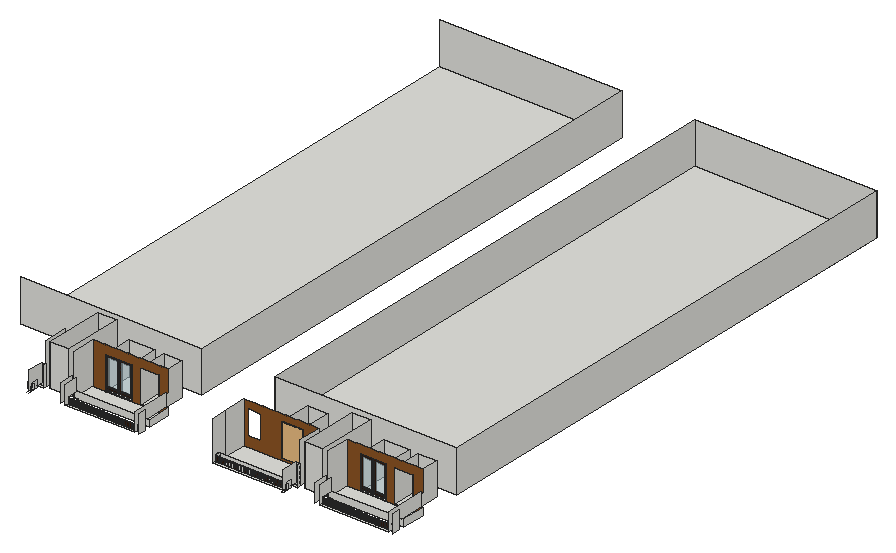
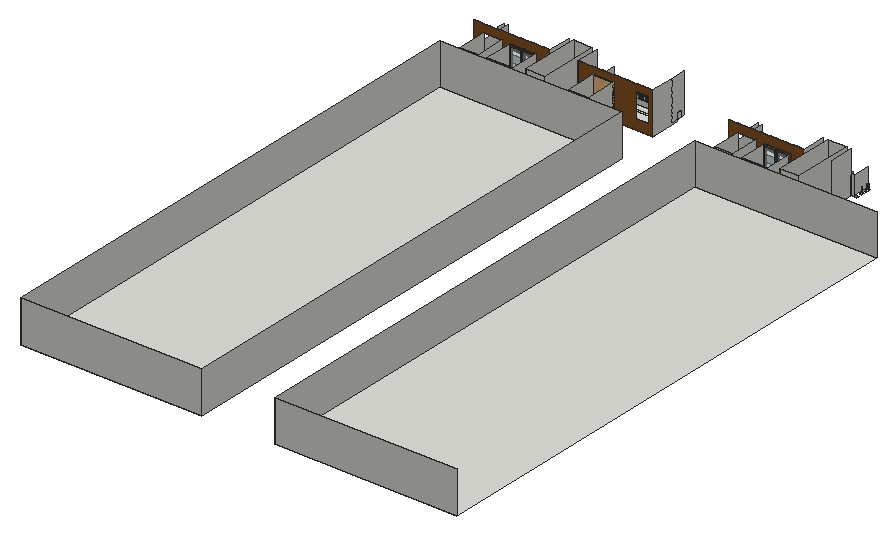
# SketchUp Ruby script. Lengths in inches.
U = 1.inch
M = Sketchup.active_model
def pt(a) = Geom::Point3d.new(a.map { |v| v * U })
def face(e, loops, mat)
  f = e.add_face(loops[0].map { |a| pt(a) })
  loops[1..].each { |l| e.add_face(l.map { |a| pt(a) }).erase! }
  f.material = f.back_material = mat if mat
  f
end
# faces: each face lists its corners as indices into pts; further lists are holes
def faces(e, pts, list, mat = nil) = list.each { |f| face(e, (f[0].is_a?(Array) ? f : [f]).map { |l| l.map { |i| pts[i] } }, mat) }
# xy, xz, yz: faces in a plane at the given z, y or x. An outline is a flat list of corners, or four numbers for a rectangle; further outlines are holes
def ring(l) = l.size == 4 ? [[l[0], l[1]], [l[2], l[1]], [l[2], l[3]], [l[0], l[3]]] : l.each_slice(2).to_a
def flat(e, list, mat, &to3) = list.each { |f| face(e, (f[0].is_a?(Array) ? f : [f]).map { |l| ring(l).map { |u, v| to3.(u, v) } }, mat) }
def xy(e, z, list, mat = nil) = flat(e, list, mat) { |x, y| [x, y, z] }
def xz(e, y, list, mat = nil) = flat(e, list, mat) { |x, z| [x, y, z] }
def yz(e, x, list, mat = nil) = flat(e, list, mat) { |y, z| [x, y, z] }
def lines(e, pts, list) = list.each { |a, b| e.add_line(pt(pts[a]), pt(pts[b])) }
# prism: a flat outline (further loops are holes) pulled along v
def prism(e, loops, v, mat = nil)
  f = face(e, loops, mat); d = Geom::Vector3d.new(v.map { |x| x * U })
  f.pushpull(f.normal.samedirection?(d) ? d.length : -d.length)
end
def box(e, o, s, mat = nil) = prism(e, [[o, [o[0] + s[0], o[1], o[2]], [o[0] + s[0], o[1] + s[1], o[2]], [o[0], o[1] + s[1], o[2]]]], [0, 0, s[2]], mat)
def at(x, y, z, deg = 0) = Geom::Transformation.translation(pt([x, y, z])) * Geom::Transformation.rotation(ORIGIN, Z_AXIS, deg.degrees)
def axes(o, x, y, z) = Geom::Transformation.new([*x, 0, *y, 0, *z, 0, *pt(o).to_a, 1])
def part(name) = M.definitions.add(name)
# library, detail: a bought-in or finely detailed component or shape, given as its bounding box
def library(name, o, s) = part(name).tap { |d| box(d.entities, o, s) }
def detail(e, o, s) = box(e.add_group.entities, o, s)
def put(e, d, t, mat = nil) = e.add_instance(d, t).tap { |i| i.material = mat if mat }
def group(e, t, mat = nil) = e.add_group.tap { |g| g.transformation = t; g.material = mat if mat }.entities
root = M.entities
M.materials.add("[Translucent Glass Safety]").color = [204, 235, 244]
M.materials["[Translucent Glass Safety]"].alpha = 0.5
M.materials.add("[Wood Floor Parquet]").color = [140, 85, 37]
M.materials.add("[Wood Veneer 01]").color = [51, 28, 15]
M.materials.add("[Wood Veneer 01]1").color = [120, 70, 37]
c1 = part("Component\#1")
xy(c1.entities,0,[[0,0,6,48]],"[Wood Veneer 01]1")
xy(c1.entities,4,[[0,4,1.8125,44],[1.8125,4,6,44]])
xy(c1.entities,80,[[0,4,1.8125,44],[1.8125,4,6,44]])
xy(c1.entities,84,[[0,0,6,48]],"[Wood Veneer 01]1")
xz(c1.entities,0,[[0,0,6,84]],"[Wood Veneer 01]1")
xz(c1.entities,4,[[0,4,1.8125,80],[1.8125,4,6,80]])
xz(c1.entities,44,[[0,4,1.8125,80],[1.8125,4,6,80]])
xz(c1.entities,48,[[0,0,6,84]],"[Wood Veneer 01]1")
yz(c1.entities,0,[[[0,0,48,84],[4,4,44,80]]],"[Wood Veneer 01]1")
yz(c1.entities,1.8125,[[4,4,44,80]],"[Translucent Glass Safety]")
yz(c1.entities,6,[[[0,0,48,84],[4,4,44,80]]],"[Wood Veneer 01]")
c2 = part("Group\#3")
put(c2.entities,c1,at(0,0,0),"[Wood Veneer 01]")
g1 = group(c2.entities,at(0,48,0),"[Wood Veneer 01]")
xy(g1,0,[[0,0,6,48]],"[Wood Veneer 01]1")
xy(g1,4,[[0,4,1.8125,44],[1.8125,4,6,44]])
xy(g1,80,[[0,4,1.8125,44],[1.8125,4,6,44]])
xy(g1,84,[[0,0,6,48]],"[Wood Veneer 01]1")
xz(g1,0,[[0,0,6,84]],"[Wood Veneer 01]1")
xz(g1,4,[[0,4,1.8125,80],[1.8125,4,6,80]])
xz(g1,44,[[0,4,1.8125,80],[1.8125,4,6,80]])
xz(g1,48,[[0,0,6,84]],"[Wood Veneer 01]1")
yz(g1,0,[[[0,0,48,84],[4,4,44,80]]],"[Wood Veneer 01]1")
yz(g1,1.8125,[[4,4,44,80]],"[Translucent Glass Safety]")
yz(g1,6,[[[0,0,48,84],[4,4,44,80]]],"[Wood Veneer 01]")
c3 = library("元件\#5",[-4.39,0,0],[5.37,35.83,90.55])
xy(root,134.6875,[[1567.3,275.15,1765.6,293.45],[1032.04,286.21,1049,293.45],[1765.6,286.21,1782.56,293.45],[1061.59,293.45,1116.3,465.02],[1130.14,293.45,1348.32,361.27],
  [1567.3,293.45,1782.56,361.27],[1795.15,293.45,1849.87,465.02],[1863.7,293.45,2081.89,361.27],[823.93,483.79,1348.32,1996.66],[1557.49,483.79,2081.89,1996.66]])
xy(root,135.5625,[[1169.05,361.27,1243.3,445.08],[1268.48,361.27,1321.23,445.08],[1902.61,361.27,1976.86,445.08],[2002.05,361.27,2054.8,445.08]])
xy(root,140.625,[[1142.89,246.64,1342.64,246.64,1342.64,256.84,1146.03,256.84,1146.03,255.72,1142.89,255.72],[1567.3,246.64,1770.48,256.84],[1876.45,246.64,2076.2,246.64,2076.2,256.84,1879.6,256.84,1879.6,255.72,1876.45,255.72],[1567.3,256.84,1770.48,256.84,1770.48,293.45,1765.6,293.45,1765.6,293.46,1567.3,293.46]])
xy(root,140.625,[[1142.89,255.72,1146.03,256.78],[1876.45,255.72,1879.6,256.78]],"[Wood Veneer 01]")
xy(root,141,[[1677.56,361.27,1736.22,452.7]])
xz(root,255.72,[[1142.89,140.625,1146.03,154.75],[1146.89,140.625,1150.03,154.75],[1150.89,140.625,1154.03,154.75],[1154.89,140.625,1158.03,154.75],[1158.89,140.625,1162.03,154.75],
  [1162.89,140.625,1166.03,154.75],[1166.89,140.625,1170.03,154.75],[1170.89,140.625,1174.03,154.75],[1174.89,140.625,1178.03,154.75],[1178.89,140.625,1182.03,154.75],
  [1182.89,140.625,1186.03,154.75],[1186.89,140.625,1190.03,154.75],[1190.89,140.625,1194.03,154.75],[1194.89,140.625,1198.03,154.75],[1198.89,140.625,1202.03,154.75],
  [1202.89,140.625,1206.03,154.75],[1206.89,140.625,1210.03,154.75],[1210.89,140.625,1214.03,154.75],[1214.89,140.625,1218.03,154.75],[1218.89,140.625,1222.03,154.75],
  [1222.89,140.625,1226.03,154.75],[1226.89,140.625,1230.03,154.75],[1230.89,140.625,1234.03,154.75],[1234.89,140.625,1238.03,154.75],[1238.89,140.625,1242.03,154.75],
  [1242.89,140.625,1246.03,154.75],[1246.89,140.625,1250.03,154.75],[1250.89,140.625,1254.03,154.75],[1254.89,140.625,1258.03,154.75],[1258.89,140.625,1262.03,154.75],
  [1262.89,140.625,1266.03,154.75],[1266.89,140.625,1270.03,154.75],[1270.89,140.625,1274.03,154.75],[1274.89,140.625,1278.03,154.75],[1278.89,140.625,1282.03,154.75],
  [1282.89,140.625,1286.03,154.75],[1286.89,140.625,1290.03,154.75],[1290.89,140.625,1294.03,154.75],[1294.89,140.625,1298.03,154.75],[1298.89,140.625,1302.03,154.75],
  [1302.89,140.625,1306.03,154.75],[1306.89,140.625,1310.03,154.75],[1310.89,140.625,1314.03,154.75],[1314.89,140.625,1318.03,154.75],[1318.89,140.625,1322.03,154.75],
  [1322.89,140.625,1326.03,154.75],[1326.89,140.625,1330.03,154.75],[1330.89,140.625,1334.03,154.75],[1334.89,140.625,1338.03,154.75],[1338.89,140.625,1342.03,154.75],
  [1342.89,140.625,1346.03,154.75],[1876.45,140.625,1879.6,154.75],[1880.45,140.625,1883.6,154.75],[1884.45,140.625,1887.6,154.75],[1888.45,140.625,1891.6,154.75],
  [1892.45,140.625,1895.6,154.75],[1896.45,140.625,1899.6,154.75],[1900.45,140.625,1903.6,154.75],[1904.45,140.625,1907.6,154.75],[1908.45,140.625,1911.6,154.75],
  [1912.45,140.625,1915.6,154.75],[1916.45,140.625,1919.6,154.75],[1920.45,140.625,1923.6,154.75],[1924.45,140.625,1927.6,154.75],[1928.45,140.625,1931.6,154.75],
  [1932.45,140.625,1935.6,154.75],[1936.45,140.625,1939.6,154.75],[1940.45,140.625,1943.6,154.75],[1944.45,140.625,1947.6,154.75],[1948.45,140.625,1951.6,154.75],
  [1952.45,140.625,1955.6,154.75],[1956.45,140.625,1959.6,154.75],[1960.45,140.625,1963.6,154.75],[1964.45,140.625,1967.6,154.75],[1968.45,140.625,1971.6,154.75],
  [1972.45,140.625,1975.6,154.75],[1976.45,140.625,1979.6,154.75],[1980.45,140.625,1983.6,154.75],[1984.45,140.625,1987.6,154.75],[1988.45,140.625,1991.6,154.75],
  [1992.45,140.625,1995.6,154.75],[1996.45,140.625,1999.6,154.75],[2000.45,140.625,2003.6,154.75],[2004.45,140.625,2007.6,154.75],[2008.45,140.625,2011.6,154.75],
  [2012.45,140.625,2015.6,154.75],[2016.45,140.625,2019.6,154.75],[2020.45,140.625,2023.6,154.75],[2024.45,140.625,2027.6,154.75],[2028.45,140.625,2031.6,154.75],
  [2032.45,140.625,2035.6,154.75],[2036.45,140.625,2039.6,154.75],[2040.45,140.625,2043.6,154.75],[2044.45,140.625,2047.6,154.75],[2048.45,140.625,2051.6,154.75],
  [2052.45,140.625,2055.6,154.75],[2056.45,140.625,2059.6,154.75],[2060.45,140.625,2063.6,154.75],[2064.45,140.625,2067.6,154.75],[2068.45,140.625,2071.6,154.75],
  [2072.45,140.625,2075.6,154.75],[2076.45,140.625,2079.6,154.75]],"[Wood Veneer 01]")
xz(root,256.78,[[1142.89,140.625,1146.03,154.75],[1876.45,140.625,1879.6,154.75]],"[Wood Veneer 01]")
xz(root,256.84,[[1026.77,140.625,1027.61,154.75],[1030.89,140.625,1031.74,154.75],[1035.02,140.625,1035.86,154.75],[1036.98,140.625,1039.14,154.75],[1039.99,140.625,1043.27,154.75],
  [1146.03,140.625,1342.64,154.75],[1342.64,140.625,1348.32,154.75],[1570.58,140.625,1571.43,154.75],[1574.7,140.625,1575.55,154.75],[1578.83,140.625,1579.68,154.75],
  [1582.95,140.625,1583.8,154.75],[1587.08,140.625,1587.93,154.75],[1591.2,140.625,1592.05,154.75],[1595.33,140.625,1596.18,154.75],[1599.45,140.625,1600.3,154.75],
  [1603.58,140.625,1604.43,154.75],[1607.7,140.625,1608.55,154.75],[1611.83,140.625,1612.68,154.75],[1615.95,140.625,1616.8,154.75],[1620.08,140.625,1620.93,154.75],
  [1624.2,140.625,1625.05,154.75],[1628.33,140.625,1629.18,154.75],[1632.45,140.625,1633.3,154.75],[1636.58,140.625,1637.43,154.75],[1640.7,140.625,1641.55,154.75],
  [1644.83,140.625,1645.68,154.75],[1648.95,140.625,1649.8,154.75],[1653.08,140.625,1653.93,154.75],[1657.2,140.625,1658.05,154.75],[1661.33,140.625,1662.18,154.75],
  [1665.45,140.625,1666.3,154.75],[1669.58,140.625,1670.43,154.75],[1673.7,140.625,1674.55,154.75],[1677.83,140.625,1678.68,154.75],[1681.95,140.625,1682.8,154.75],
  [1686.08,140.625,1686.93,154.75],[1690.2,140.625,1691.05,154.75],[1694.33,140.625,1695.18,154.75],[1698.45,140.625,1699.3,154.75],[1702.58,140.625,1703.43,154.75],
  [1706.7,140.625,1707.55,154.75],[1710.83,140.625,1711.68,154.75],[1714.95,140.625,1715.8,154.75],[1719.08,140.625,1719.93,154.75],[1723.2,140.625,1724.05,154.75],
  [1727.33,140.625,1728.18,154.75],[1731.45,140.625,1732.3,154.75],[1735.58,140.625,1736.43,154.75],[1739.7,140.625,1740.55,154.75],[1743.83,140.625,1744.68,154.75],
  [1747.95,140.625,1748.8,154.75],[1752.08,140.625,1752.93,154.75],[1756.2,140.625,1757.05,154.75],[1760.33,140.625,1761.18,154.75],[1764.45,140.625,1765.3,154.75],
  [1768.58,140.625,1769.43,154.75],[1770.54,140.625,1772.7,154.75],[1773.55,140.625,1776.83,154.75],[1879.6,140.625,2076.2,154.75],[2076.2,140.625,2081.89,154.75]])
xz(root,256.84,[[1027.61,140.625,1030.89,154.75],[1031.74,140.625,1035.02,154.75],[1035.86,140.625,1036.98,154.75],[1567.3,140.625,1570.58,154.75],[1571.43,140.625,1574.7,154.75],
  [1575.55,140.625,1578.83,154.75],[1579.68,140.625,1582.95,154.75],[1583.8,140.625,1587.08,154.75],[1587.93,140.625,1591.2,154.75],[1592.05,140.625,1595.33,154.75],
  [1596.18,140.625,1599.45,154.75],[1600.3,140.625,1603.58,154.75],[1604.43,140.625,1607.7,154.75],[1608.55,140.625,1611.83,154.75],[1612.68,140.625,1615.95,154.75],
  [1616.8,140.625,1620.08,154.75],[1620.93,140.625,1624.2,154.75],[1625.05,140.625,1628.33,154.75],[1629.18,140.625,1632.45,154.75],[1633.3,140.625,1636.58,154.75],
  [1637.43,140.625,1640.7,154.75],[1641.55,140.625,1644.83,154.75],[1645.68,140.625,1648.95,154.75],[1649.8,140.625,1653.08,154.75],[1653.93,140.625,1657.2,154.75],
  [1658.05,140.625,1661.33,154.75],[1662.18,140.625,1665.45,154.75],[1666.3,140.625,1669.58,154.75],[1670.43,140.625,1673.7,154.75],[1674.55,140.625,1677.83,154.75],
  [1678.68,140.625,1681.95,154.75],[1682.8,140.625,1686.08,154.75],[1686.93,140.625,1690.2,154.75],[1691.05,140.625,1694.33,154.75],[1695.18,140.625,1698.45,154.75],
  [1699.3,140.625,1702.58,154.75],[1703.43,140.625,1706.7,154.75],[1707.55,140.625,1710.83,154.75],[1711.68,140.625,1714.95,154.75],[1715.8,140.625,1719.08,154.75],
  [1719.93,140.625,1723.2,154.75],[1724.05,140.625,1727.33,154.75],[1728.18,140.625,1731.45,154.75],[1732.3,140.625,1735.58,154.75],[1736.43,140.625,1739.7,154.75],
  [1740.55,140.625,1743.83,154.75],[1744.68,140.625,1747.95,154.75],[1748.8,140.625,1752.08,154.75],[1752.93,140.625,1756.2,154.75],[1757.05,140.625,1760.33,154.75],
  [1761.18,140.625,1764.45,154.75],[1765.3,140.625,1768.58,154.75],[1769.43,140.625,1770.54,154.75]],"[Wood Veneer 01]")
xz(root,266.43,[[1348.32,140.625,1355.5625,154.75],[2081.89,140.625,2089.125,154.75]])
xz(root,275.15,[[1032.04,134.6875,1036.98,154.75],[1567.3,134.6875,1765.6,154.75],[1765.6,134.6875,1770.54,154.75]])
xz(root,293.45,[[1032.04,134.6875,1032.04,140.625,1036.91,140.625,1036.91,193,1049,193,1049,134.6875],[1061.59,134.6875,1116.3,254.6875],[1130.14,134.6875,1348.32,154.75],[1765.6,134.6875,1765.6,140.625,1770.48,140.625,1770.48,193,1782.56,193,1782.56,134.6875],[1795.15,134.6875,1849.87,254.6875],
  [1863.7,134.6875,2081.89,154.75]])
xz(root,361.27,[[1169.05,134.6875,1243.3,135.5625],[1268.48,134.6875,1321.23,135.5625],[1902.61,134.6875,1976.86,135.5625],[2002.05,134.6875,2054.8,135.5625]])
xz(root,361.27,[[1130.14,134.6875,1169.05,134.6875,1169.05,230.0625,1243.3,230.0625,1243.3,134.6875,1268.48,134.6875,1268.48,230.125,1321.23,230.125,1321.23,134.6875,1348.32,134.6875,1348.32,154.75,1342.64,154.75,1342.64,193,1348.32,193,1348.32,253.9375,1346.14,253.9375,1346.14,254.6875,1344.52,254.6875,1344.52,253.9375,1340.14,253.9375,1340.14,254.6875,1338.52,254.6875,1338.52,253.9375,1334.14,253.9375,1334.14,254.6875,1332.52,254.6875,1332.52,253.9375,1328.14,253.9375,1328.14,254.6875,1326.52,254.6875,1326.52,253.9375,1322.14,253.9375,1322.14,254.6875,1320.52,254.6875,1320.52,253.9375,1316.14,253.9375,1316.14,254.6875,1314.52,254.6875,1314.52,253.9375,1310.14,253.9375,1310.14,254.6875,1308.52,254.6875,1308.52,253.9375,1304.14,253.9375,1304.14,254.6875,1302.52,254.6875,1302.52,253.9375,1298.14,253.9375,1298.14,254.6875,1296.52,254.6875,1296.52,253.9375,1292.14,253.9375,1292.14,254.6875,1290.52,254.6875,1290.52,253.9375,1286.14,253.9375,1286.14,254.6875,1284.52,254.6875,1284.52,253.9375,1280.14,253.9375,1280.14,254.6875,1278.52,254.6875,1278.52,253.9375,1274.14,253.9375,1274.14,254.6875,1272.52,254.6875,1272.52,253.9375,1268.14,253.9375,1268.14,254.6875,1266.52,254.6875,1266.52,253.9375,1262.14,253.9375,1262.14,254.6875,1260.52,254.6875,1260.52,253.9375,1256.14,253.9375,1256.14,254.6875,1254.52,254.6875,1254.52,253.9375,1250.14,253.9375,1250.14,254.6875,1248.52,254.6875,1248.52,253.9375,1244.14,253.9375,1244.14,254.6875,1242.52,254.6875,1242.52,253.9375,1238.14,253.9375,1238.14,254.6875,1236.52,254.6875,1236.52,253.9375,1232.14,253.9375,1232.14,254.6875,1230.52,254.6875,1230.52,253.9375,1226.14,253.9375,1226.14,254.6875,1224.52,254.6875,1224.52,253.9375,1220.14,253.9375,1220.14,254.6875,1218.52,254.6875,1218.52,253.9375,1214.14,253.9375,1214.14,254.6875,1212.52,254.6875,1212.52,253.9375,1208.14,253.9375,1208.14,254.6875,1206.52,254.6875,1206.52,253.9375,1202.14,253.9375,1202.14,254.6875,1200.52,254.6875,1200.52,253.9375,1196.14,253.9375,1196.14,254.6875,1194.52,254.6875,1194.52,253.9375,1190.14,253.9375,1190.14,254.6875,1188.52,254.6875,1188.52,253.9375,1184.14,253.9375,1184.14,254.6875,1182.52,254.6875,1182.52,253.9375,1178.14,253.9375,1178.14,254.6875,1176.52,254.6875,1176.52,253.9375,1172.14,253.9375,1172.14,254.6875,1170.52,254.6875,1170.52,253.9375,1166.14,253.9375,1166.14,254.6875,1164.52,254.6875,1164.52,253.9375,1160.14,253.9375,1160.14,254.6875,1158.52,254.6875,1158.52,253.9375,1154.14,253.9375,1154.14,254.6875,1152.52,254.6875,1152.52,253.9375,1148.14,253.9375,1148.14,254.6875,1146.52,254.6875,1146.52,253.9375,1142.14,253.9375,1142.14,254.6875,1140.52,254.6875,1140.52,253.9375,1136.14,253.9375,1136.14,254.6875,1134.52,254.6875,1134.52,253.9375,1130.14,253.9375],[[1567.3,134.6875,1782.56,134.6875,1782.56,253.5625,1777.81,253.5625,1777.81,254.6875,1776.56,254.6875,1776.56,253.5625,1771.81,253.5625,1771.81,254.6875,1770.56,254.6875,1770.56,253.5625,1765.81,253.5625,1765.81,254.6875,1764.56,254.6875,1764.56,253.5625,1759.81,253.5625,1759.81,254.6875,1758.56,254.6875,1758.56,253.5625,1753.81,253.5625,1753.81,254.6875,1752.56,254.6875,1752.56,253.5625,1747.81,253.5625,1747.81,254.6875,1746.56,254.6875,1746.56,253.5625,1741.81,253.5625,1741.81,254.6875,1740.56,254.6875,1740.56,253.5625,1735.81,253.5625,1735.81,254.6875,1734.56,254.6875,1734.56,253.5625,1729.81,253.5625,1729.81,254.6875,1728.56,254.6875,1728.56,253.5625,1723.81,253.5625,1723.81,254.6875,1722.56,254.6875,1722.56,253.875,1717.81,253.875,1717.81,254.6875,1716.56,254.6875,1716.56,253.875,1711.81,253.875,1711.81,254.6875,1710.56,254.6875,1710.56,253.9375,1705.81,253.9375,1705.81,254.6875,1704.56,254.6875,1704.56,253.9375,1699.81,253.9375,1699.81,254.6875,1698.56,254.6875,1698.56,253.9375,1693.81,253.9375,1693.81,254.6875,1692.56,254.6875,1692.56,253.9375,1687.81,253.9375,1687.81,254.6875,1686.56,254.6875,1686.56,253.9375,1681.81,253.9375,1681.81,254.6875,1680.56,254.6875,1680.56,253.9375,1675.81,253.9375,1675.81,254.6875,1674.56,254.6875,1674.56,253.9375,1669.81,253.9375,1669.81,254.6875,1668.56,254.6875,1668.56,253.9375,1663.81,253.9375,1663.81,254.6875,1662.56,254.6875,1662.56,253.9375,1657.81,253.9375,1657.81,254.6875,1656.56,254.6875,1656.56,253.9375,1651.81,253.9375,1651.81,254.6875,1650.56,254.6875,1650.56,253.9375,1645.81,253.9375,1645.81,254.6875,1644.56,254.6875,1644.56,253.9375,1639.81,253.9375,1639.81,254.6875,1638.56,254.6875,1638.56,253.9375,1633.81,253.9375,1633.81,254.6875,1632.56,254.6875,1632.56,253.9375,1627.81,253.9375,1627.81,254.6875,1626.56,254.6875,1626.56,253.9375,1621.81,253.9375,1621.81,254.6875,1620.56,254.6875,1620.56,253.9375,1615.81,253.9375,1615.81,254.6875,1614.56,254.6875,1614.56,253.9375,1609.81,253.9375,1609.81,254.6875,1608.56,254.6875,1608.56,253.9375,1603.81,253.9375,1603.81,254.6875,1602.56,254.6875,1602.56,253.9375,1597.81,253.9375,1597.81,254.6875,1596.56,254.6875,1596.56,253.9375,1591.81,253.9375,1591.81,254.6875,1590.56,254.6875,1590.56,253.9375,1585.81,253.9375,1585.81,254.6875,1584.56,254.6875,1584.56,253.9375,1579.81,253.9375,1579.81,254.6875,1567.3,254.6875],[1677.56,141,1736.22,235.92],[1579.05,162.74,1616.36,234.87]],[1863.7,134.6875,1902.61,134.6875,1902.61,230.0625,1976.86,230.0625,1976.86,134.6875,2002.05,134.6875,2002.05,230.125,2054.8,230.125,2054.8,134.6875,2081.89,134.6875,2081.89,154.75,2076.2,154.75,2076.2,193,2081.89,193,2081.89,253.9375,2079.7,253.9375,2079.7,254.6875,2078.08,254.6875,2078.08,253.9375,2073.7,253.9375,2073.7,254.6875,2072.08,254.6875,2072.08,253.9375,2067.7,253.9375,2067.7,254.6875,2066.08,254.6875,2066.08,253.9375,2061.7,253.9375,2061.7,254.6875,2060.08,254.6875,2060.08,253.9375,2055.7,253.9375,2055.7,254.6875,2054.08,254.6875,2054.08,253.9375,2049.7,253.9375,2049.7,254.6875,2048.08,254.6875,2048.08,253.9375,2043.7,253.9375,2043.7,254.6875,2042.08,254.6875,2042.08,253.9375,2037.7,253.9375,2037.7,254.6875,2036.08,254.6875,2036.08,253.9375,2031.7,253.9375,2031.7,254.6875,2030.08,254.6875,2030.08,253.9375,2025.7,253.9375,2025.7,254.6875,2024.08,254.6875,2024.08,253.9375,2019.7,253.9375,2019.7,254.6875,2018.08,254.6875,2018.08,253.9375,2013.7,253.9375,2013.7,254.6875,2012.08,254.6875,2012.08,253.9375,2007.7,253.9375,2007.7,254.6875,2006.08,254.6875,2006.08,253.9375,2001.7,253.9375,2001.7,254.6875,2000.08,254.6875,2000.08,253.9375,1995.7,253.9375,1995.7,254.6875,1994.08,254.6875,1994.08,253.9375,1989.7,253.9375,1989.7,254.6875,1988.08,254.6875,1988.08,253.9375,1983.7,253.9375,1983.7,254.6875,1982.08,254.6875,1982.08,253.9375,1977.7,253.9375,1977.7,254.6875,1976.08,254.6875,1976.08,253.9375,1971.7,253.9375,1971.7,254.6875,1970.08,254.6875,1970.08,253.9375,1965.7,253.9375,1965.7,254.6875,1964.08,254.6875,1964.08,253.9375,1959.7,253.9375,1959.7,254.6875,1958.08,254.6875,1958.08,253.9375,1953.7,253.9375,1953.7,254.6875,1952.08,254.6875,1952.08,253.9375,1947.7,253.9375,1947.7,254.6875,1946.08,254.6875,1946.08,253.9375,1941.7,253.9375,1941.7,254.6875,1940.08,254.6875,1940.08,253.9375,1935.7,253.9375,1935.7,254.6875,1934.08,254.6875,1934.08,253.9375,1929.7,253.9375,1929.7,254.6875,1928.08,254.6875,1928.08,253.9375,1923.7,253.9375,1923.7,254.6875,1922.08,254.6875,1922.08,253.9375,1917.7,253.9375,1917.7,254.6875,1916.08,254.6875,1916.08,253.9375,1911.7,253.9375,1911.7,254.6875,1910.08,254.6875,1910.08,253.9375,1905.7,253.9375,1905.7,254.6875,1904.08,254.6875,1904.08,253.9375,1899.7,253.9375,1899.7,254.6875,1898.08,254.6875,1898.08,253.9375,1893.7,253.9375,1893.7,254.6875,1892.08,254.6875,1892.08,253.9375,1887.7,253.9375,1887.7,254.6875,1886.08,254.6875,1886.08,253.9375,1881.7,253.9375,1881.7,254.6875,1880.08,254.6875,1880.08,253.9375,1875.7,253.9375,1875.7,254.6875,1874.08,254.6875,1874.08,253.9375,1869.7,253.9375,1869.7,254.6875,1868.08,254.6875,1868.08,253.9375,1863.7,253.9375]],"[Wood Floor Parquet]")
xz(root,445.08,[[1169.05,135.5625,1243.3,230.0625],[1268.48,135.5625,1321.23,230.125],[1902.61,135.5625,1976.86,230.0625],[2002.05,135.5625,2054.8,230.125]])
xz(root,452.7,[[1677.56,141,1736.22,235.92]])
xz(root,465.02,[[1061.59,134.6875,1116.3,254.6875],[1795.15,134.6875,1849.87,254.6875]])
xz(root,483.79,[[823.93,134.6875,1348.32,254.6875],[1557.49,134.6875,2081.89,254.6875]])
xz(root,1996.66,[[823.93,134.6875,1348.32,254.6875],[1557.49,134.6875,2081.89,254.6875]])
yz(root,1036.91,[[246.64,140.625,293.45,193]])
yz(root,1036.98,[[256.84,134.6875,275.15,154.75]])
yz(root,1049,[[286.21,134.6875,293.45,193],[293.45,134.6875,293.46,193],[293.46,134.6875,293.46,193,293.45,193,293.45,253.5625,361.27,253.5625,361.27,134.6875]])
yz(root,1061.59,[[293.45,134.6875,465.02,254.6875]])
yz(root,1116.3,[[293.45,134.6875,465.02,254.6875]])
yz(root,1130.14,[[293.45,134.6875,361.27,253.9375],[246.64,141.6875,286.21,193]])
yz(root,1142.89,[[246.64,140.625,255.72,140.625,255.72,154.75,254.22,154.75,254.22,156.9375,286.21,156.9375,286.21,193,246.64,193]])
yz(root,1142.89,[[255.72,140.625,256.78,154.75]],"[Wood Veneer 01]")
yz(root,1146.03,[[255.72,140.625,256.78,154.75],[256.78,140.625,256.84,154.75]],"[Wood Veneer 01]")
yz(root,1150.03,[[255.72,140.625,256.78,154.75]],"[Wood Veneer 01]")
yz(root,1154.03,[[255.72,140.625,256.78,154.75]],"[Wood Veneer 01]")
yz(root,1158.03,[[255.72,140.625,256.78,154.75]],"[Wood Veneer 01]")
yz(root,1162.03,[[255.72,140.625,256.78,154.75]],"[Wood Veneer 01]")
yz(root,1166.03,[[255.72,140.625,256.78,154.75]],"[Wood Veneer 01]")
yz(root,1169.05,[[361.27,135.5625,445.08,230.0625]])
yz(root,1170.03,[[255.72,140.625,256.78,154.75]],"[Wood Veneer 01]")
yz(root,1174.03,[[255.72,140.625,256.78,154.75]],"[Wood Veneer 01]")
yz(root,1178.03,[[255.72,140.625,256.78,154.75]],"[Wood Veneer 01]")
yz(root,1182.03,[[255.72,140.625,256.78,154.75]],"[Wood Veneer 01]")
yz(root,1186.03,[[255.72,140.625,256.78,154.75]],"[Wood Veneer 01]")
yz(root,1190.03,[[255.72,140.625,256.78,154.75]],"[Wood Veneer 01]")
yz(root,1194.03,[[255.72,140.625,256.78,154.75]],"[Wood Veneer 01]")
yz(root,1198.03,[[255.72,140.625,256.78,154.75]],"[Wood Veneer 01]")
yz(root,1202.03,[[255.72,140.625,256.78,154.75]],"[Wood Veneer 01]")
yz(root,1206.03,[[255.72,140.625,256.78,154.75]],"[Wood Veneer 01]")
yz(root,1210.03,[[255.72,140.625,256.78,154.75]],"[Wood Veneer 01]")
yz(root,1214.03,[[255.72,140.625,256.78,154.75]],"[Wood Veneer 01]")
yz(root,1218.03,[[255.72,140.625,256.78,154.75]],"[Wood Veneer 01]")
yz(root,1222.03,[[255.72,140.625,256.78,154.75]],"[Wood Veneer 01]")
yz(root,1226.03,[[255.72,140.625,256.78,154.75]],"[Wood Veneer 01]")
yz(root,1230.03,[[255.72,140.625,256.78,154.75]],"[Wood Veneer 01]")
yz(root,1234.03,[[255.72,140.625,256.78,154.75]],"[Wood Veneer 01]")
yz(root,1238.03,[[255.72,140.625,256.78,154.75]],"[Wood Veneer 01]")
yz(root,1242.03,[[255.72,140.625,256.78,154.75]],"[Wood Veneer 01]")
yz(root,1243.3,[[361.27,135.5625,445.08,230.0625]])
yz(root,1246.03,[[255.72,140.625,256.78,154.75]],"[Wood Veneer 01]")
yz(root,1250.03,[[255.72,140.625,256.78,154.75]],"[Wood Veneer 01]")
yz(root,1254.03,[[255.72,140.625,256.78,154.75]],"[Wood Veneer 01]")
yz(root,1258.03,[[255.72,140.625,256.78,154.75]],"[Wood Veneer 01]")
yz(root,1262.03,[[255.72,140.625,256.78,154.75]],"[Wood Veneer 01]")
yz(root,1266.03,[[255.72,140.625,256.78,154.75]],"[Wood Veneer 01]")
yz(root,1268.48,[[361.27,135.5625,445.08,230.125]])
yz(root,1270.03,[[255.72,140.625,256.78,154.75]],"[Wood Veneer 01]")
yz(root,1274.03,[[255.72,140.625,256.78,154.75]],"[Wood Veneer 01]")
yz(root,1278.03,[[255.72,140.625,256.78,154.75]],"[Wood Veneer 01]")
yz(root,1282.03,[[255.72,140.625,256.78,154.75]],"[Wood Veneer 01]")
yz(root,1286.03,[[255.72,140.625,256.78,154.75]],"[Wood Veneer 01]")
yz(root,1290.03,[[255.72,140.625,256.78,154.75]],"[Wood Veneer 01]")
yz(root,1294.03,[[255.72,140.625,256.78,154.75]],"[Wood Veneer 01]")
yz(root,1298.03,[[255.72,140.625,256.78,154.75]],"[Wood Veneer 01]")
yz(root,1302.03,[[255.72,140.625,256.78,154.75]],"[Wood Veneer 01]")
yz(root,1306.03,[[255.72,140.625,256.78,154.75]],"[Wood Veneer 01]")
yz(root,1321.23,[[361.27,135.5625,445.08,230.125]])
yz(root,1342.64,[[246.64,140.625,246.64,193,361.27,193,361.27,154.75,293.45,154.75,293.45,156.9375,254.22,156.9375,254.22,154.75,256.84,154.75,256.84,140.625]])
yz(root,1348.32,[[293.45,134.6875,361.27,154.75],[483.79,134.6875,1996.66,254.6875],[256.84,140.625,266.43,154.75]])
yz(root,1355.5625,[[246.64,140.625,266.43,193]])
yz(root,1557.49,[[483.79,134.6875,1996.66,254.6875]])
yz(root,1567.3,[[275.15,134.6875,361.27,134.6875,361.27,254.6875,293.46,254.6875,293.46,140.625,275.15,140.625],[246.64,140.625,256.84,140.625,256.84,154.75,254.22,154.75,254.22,158.1875,275.15,158.1875,275.15,140.625,293.46,140.625,293.46,254.6875,246.64,254.6875],[256.84,140.625,275.15,154.75]])
yz(root,1677.56,[[361.27,141,452.7,235.92]])
yz(root,1736.22,[[361.27,141,452.7,235.92]])
yz(root,1770.48,[[246.64,140.625,293.45,193]])
yz(root,1770.54,[[256.84,134.6875,275.15,154.75]])
yz(root,1782.56,[[286.21,134.6875,293.45,193],[293.45,134.6875,293.46,193],[293.46,134.6875,293.46,193,293.45,193,293.45,253.5625,361.27,253.5625,361.27,134.6875]])
yz(root,1795.15,[[293.45,134.6875,465.02,254.6875]])
yz(root,1849.87,[[293.45,134.6875,465.02,254.6875]])
yz(root,1863.7,[[293.45,134.6875,361.27,253.9375],[246.64,141.6875,286.21,193]])
yz(root,1876.45,[[246.64,140.625,255.72,140.625,255.72,154.75,254.22,154.75,254.22,156.9375,286.21,156.9375,286.21,193,246.64,193]])
yz(root,1876.45,[[255.72,140.625,256.78,154.75]],"[Wood Veneer 01]")
yz(root,1879.6,[[255.72,140.625,256.78,154.75],[256.78,140.625,256.84,154.75]],"[Wood Veneer 01]")
yz(root,1883.6,[[255.72,140.625,256.78,154.75]],"[Wood Veneer 01]")
yz(root,1887.6,[[255.72,140.625,256.78,154.75]],"[Wood Veneer 01]")
yz(root,1891.6,[[255.72,140.625,256.78,154.75]],"[Wood Veneer 01]")
yz(root,1895.6,[[255.72,140.625,256.78,154.75]],"[Wood Veneer 01]")
yz(root,1899.6,[[255.72,140.625,256.78,154.75]],"[Wood Veneer 01]")
yz(root,1902.61,[[361.27,135.5625,445.08,230.0625]])
yz(root,1903.6,[[255.72,140.625,256.78,154.75]],"[Wood Veneer 01]")
yz(root,1907.6,[[255.72,140.625,256.78,154.75]],"[Wood Veneer 01]")
yz(root,1911.6,[[255.72,140.625,256.78,154.75]],"[Wood Veneer 01]")
yz(root,1915.6,[[255.72,140.625,256.78,154.75]],"[Wood Veneer 01]")
yz(root,1919.6,[[255.72,140.625,256.78,154.75]],"[Wood Veneer 01]")
yz(root,1923.6,[[255.72,140.625,256.78,154.75]],"[Wood Veneer 01]")
yz(root,1927.6,[[255.72,140.625,256.78,154.75]],"[Wood Veneer 01]")
yz(root,1931.6,[[255.72,140.625,256.78,154.75]],"[Wood Veneer 01]")
yz(root,1935.6,[[255.72,140.625,256.78,154.75]],"[Wood Veneer 01]")
yz(root,1939.6,[[255.72,140.625,256.78,154.75]],"[Wood Veneer 01]")
yz(root,1943.6,[[255.72,140.625,256.78,154.75]],"[Wood Veneer 01]")
yz(root,1947.6,[[255.72,140.625,256.78,154.75]],"[Wood Veneer 01]")
yz(root,1951.6,[[255.72,140.625,256.78,154.75]],"[Wood Veneer 01]")
yz(root,1955.6,[[255.72,140.625,256.78,154.75]],"[Wood Veneer 01]")
yz(root,1959.6,[[255.72,140.625,256.78,154.75]],"[Wood Veneer 01]")
yz(root,1963.6,[[255.72,140.625,256.78,154.75]],"[Wood Veneer 01]")
yz(root,1967.6,[[255.72,140.625,256.78,154.75]],"[Wood Veneer 01]")
yz(root,1971.6,[[255.72,140.625,256.78,154.75]],"[Wood Veneer 01]")
yz(root,1975.6,[[255.72,140.625,256.78,154.75]],"[Wood Veneer 01]")
yz(root,1976.86,[[361.27,135.5625,445.08,230.0625]])
yz(root,1979.6,[[255.72,140.625,256.78,154.75]],"[Wood Veneer 01]")
yz(root,1983.6,[[255.72,140.625,256.78,154.75]],"[Wood Veneer 01]")
yz(root,1987.6,[[255.72,140.625,256.78,154.75]],"[Wood Veneer 01]")
yz(root,1991.6,[[255.72,140.625,256.78,154.75]],"[Wood Veneer 01]")
yz(root,1995.6,[[255.72,140.625,256.78,154.75]],"[Wood Veneer 01]")
yz(root,1999.6,[[255.72,140.625,256.78,154.75]],"[Wood Veneer 01]")
yz(root,2002.05,[[361.27,135.5625,445.08,230.125]])
yz(root,2003.6,[[255.72,140.625,256.78,154.75]],"[Wood Veneer 01]")
yz(root,2007.6,[[255.72,140.625,256.78,154.75]],"[Wood Veneer 01]")
yz(root,2011.6,[[255.72,140.625,256.78,154.75]],"[Wood Veneer 01]")
yz(root,2015.6,[[255.72,140.625,256.78,154.75]],"[Wood Veneer 01]")
yz(root,2019.6,[[255.72,140.625,256.78,154.75]],"[Wood Veneer 01]")
yz(root,2023.6,[[255.72,140.625,256.78,154.75]],"[Wood Veneer 01]")
yz(root,2027.6,[[255.72,140.625,256.78,154.75]],"[Wood Veneer 01]")
yz(root,2031.6,[[255.72,140.625,256.78,154.75]],"[Wood Veneer 01]")
yz(root,2035.6,[[255.72,140.625,256.78,154.75]],"[Wood Veneer 01]")
yz(root,2039.6,[[255.72,140.625,256.78,154.75]],"[Wood Veneer 01]")
yz(root,2054.8,[[361.27,135.5625,445.08,230.125]])
yz(root,2076.2,[[246.64,140.625,246.64,193,361.27,193,361.27,154.75,293.45,154.75,293.45,156.9375,254.22,156.9375,254.22,154.75,256.84,154.75,256.84,140.625]])
yz(root,2081.89,[[293.45,134.6875,361.27,154.75],[483.79,134.6875,1996.66,254.6875],[256.84,140.625,266.43,154.75]])
yz(root,2089.125,[[246.64,140.625,266.43,193]])
p = [[1036.98,256.84,134.6875],[1036.98,246.64,134.6875],[1032.04,275.15,134.6875],[1032.04,246.64,134.6875],[1149.2,266.43,141.6875],[1149.2,286.21,141.6875],
  [1130.14,286.21,141.6875],[1032.04,275.15,140.625],[1036.91,275.15,140.625],[1310.03,256.78,140.625],[1310.03,256.78,154.75],[1310.03,255.72,140.625],
  [1314.03,256.78,140.625],[1314.03,256.78,154.75],[1314.03,255.72,140.625],[1318.03,256.78,140.625],[1318.03,256.78,154.75],[1318.03,255.72,140.625],
  [1322.03,256.78,140.625],[1322.03,256.78,154.75],[1322.03,255.72,140.625],[1326.03,256.78,140.625],[1326.03,256.78,154.75],[1326.03,255.72,140.625],
  [1330.03,256.78,140.625],[1330.03,256.78,154.75],[1330.03,255.72,140.625],[1334.03,256.78,140.625],[1334.03,256.78,154.75],[1334.03,255.72,140.625],
  [1338.03,256.78,140.625],[1338.03,256.78,154.75],[1338.03,255.72,140.625],[1342.03,256.78,140.625],[1342.03,256.78,154.75],[1342.03,255.72,140.625],
  [1346.03,256.78,140.625],[1346.03,256.78,154.75],[1346.03,255.72,140.625],[1765.6,275.15,134.6875],[1765.6,246.64,134.6875],[1765.6,275.15,140.625],
  [1770.48,275.15,140.625],[1770.54,256.84,134.6875],[1770.54,246.64,134.6875],[1863.7,286.21,141.6875],[1882.76,286.21,141.6875],[1882.76,266.43,141.6875],
  [2047.6,256.78,140.625],[2047.6,256.78,154.75],[2055.6,256.78,140.625],[2055.6,256.78,154.75],[2043.6,256.78,140.625],[2043.6,256.78,154.75],
  [2047.6,255.72,140.625],[2055.6,255.72,140.625],[2051.6,256.78,140.625],[2051.6,255.72,140.625],[2059.6,256.78,140.625],[2059.6,256.78,154.75],
  [2043.6,255.72,140.625],[2059.6,255.72,140.625],[2063.6,256.78,140.625],[2063.6,256.78,154.75],[2063.6,255.72,140.625],[2067.6,256.78,140.625],
  [2067.6,256.78,154.75],[2051.6,256.78,154.75],[2067.6,255.72,140.625],[2071.6,256.78,140.625],[2071.6,256.78,154.75],[2071.6,255.72,140.625],
  [2075.6,256.78,140.625],[2075.6,256.78,154.75],[2075.6,255.72,140.625],[2079.6,256.78,140.625],[2079.6,256.78,154.75],[2079.6,255.72,140.625]]
lines(root,p,[[0,1],[2,3],[4,5],[6,5],[7,8],[9,10],[9,11],[12,13],[12,14],[15,16],[15,17],[18,19],
  [18,20],[21,22],[21,23],[24,25],[24,26],[27,28],[27,29],[30,31],[30,32],[33,34],[33,35],[36,37],
  [36,38],[39,40],[41,42],[43,44],[45,46],[47,46],[48,49],[50,51],[52,53],[48,54],[50,55],[56,57],
  [58,59],[52,60],[58,61],[62,63],[62,64],[65,66],[56,67],[65,68],[69,70],[69,71],[72,73],[72,74],
  [75,76],[75,77]])
put(root,c2,axes([1169.05,367.27,141.22],[0,-1,0],[0.77344,0,0],[0,0,1.0577]))
put(root,c3,axes([1677.56,361.64,141],[0,-1,0],[1.63746,0,0],[0,0,1.04827]))
put(root,c2,axes([1902.61,367.27,141.22],[0,-1,0],[0.77344,0,0],[0,0,1.0577]))
